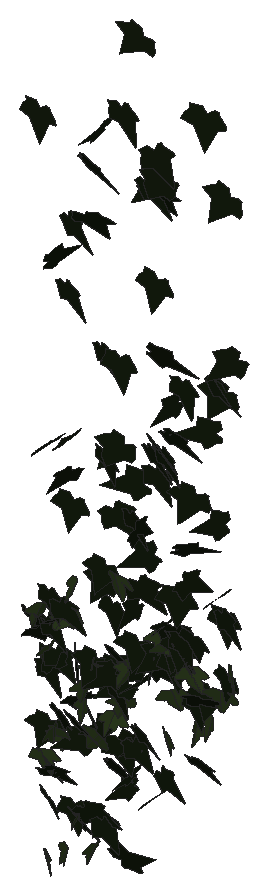
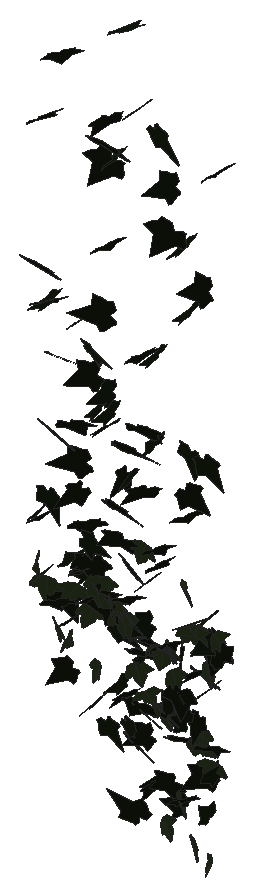
# SketchUp Ruby script. Lengths in inches.
U = 1.inch
M = Sketchup.active_model
def pt(a) = Geom::Point3d.new(a.map { |v| v * U })
def face(e, loops, mat)
  f = e.add_face(loops[0].map { |a| pt(a) })
  loops[1..].each { |l| e.add_face(l.map { |a| pt(a) }).erase! }
  f.material = f.back_material = mat if mat
  f
end
# faces: each face lists its corners as indices into pts; further lists are holes
def faces(e, pts, list, mat = nil) = list.each { |f| face(e, (f[0].is_a?(Array) ? f : [f]).map { |l| l.map { |i| pts[i] } }, mat) }
# xy, xz, yz: faces in a plane at the given z, y or x. An outline is a flat list of corners, or four numbers for a rectangle; further outlines are holes
def ring(l) = l.size == 4 ? [[l[0], l[1]], [l[2], l[1]], [l[2], l[3]], [l[0], l[3]]] : l.each_slice(2).to_a
def flat(e, list, mat, &to3) = list.each { |f| face(e, (f[0].is_a?(Array) ? f : [f]).map { |l| ring(l).map { |u, v| to3.(u, v) } }, mat) }
def xy(e, z, list, mat = nil) = flat(e, list, mat) { |x, y| [x, y, z] }
def xz(e, y, list, mat = nil) = flat(e, list, mat) { |x, z| [x, y, z] }
def yz(e, x, list, mat = nil) = flat(e, list, mat) { |y, z| [x, y, z] }
def lines(e, pts, list) = list.each { |a, b| e.add_line(pt(pts[a]), pt(pts[b])) }
# prism: a flat outline (further loops are holes) pulled along v
def prism(e, loops, v, mat = nil)
  f = face(e, loops, mat); d = Geom::Vector3d.new(v.map { |x| x * U })
  f.pushpull(f.normal.samedirection?(d) ? d.length : -d.length)
end
def box(e, o, s, mat = nil) = prism(e, [[o, [o[0] + s[0], o[1], o[2]], [o[0] + s[0], o[1] + s[1], o[2]], [o[0], o[1] + s[1], o[2]]]], [0, 0, s[2]], mat)
def at(x, y, z, deg = 0) = Geom::Transformation.translation(pt([x, y, z])) * Geom::Transformation.rotation(ORIGIN, Z_AXIS, deg.degrees)
def axes(o, x, y, z) = Geom::Transformation.new([*x, 0, *y, 0, *z, 0, *pt(o).to_a, 1])
def part(name) = M.definitions.add(name)
# library, detail: a bought-in or finely detailed component or shape, given as its bounding box
def library(name, o, s) = part(name).tap { |d| box(d.entities, o, s) }
def detail(e, o, s) = box(e.add_group.entities, o, s)
def put(e, d, t, mat = nil) = e.add_instance(d, t).tap { |i| i.material = mat if mat }
def group(e, t, mat = nil) = e.add_group.tap { |g| g.transformation = t; g.material = mat if mat }.entities
root = M.entities
M.materials.add("1026 AP 7946 SUNNY SIDE UP").color = [254, 231, 186]
M.materials.add("efeu1").color = [18, 25, 13]
M.materials.add("efeu2").color = [43, 57, 29]
c1 = part("ivyleaf_9")
p = [[1.54,2.16,1.25],[1.36,2.04,1.19],[-0.21,0.99,0.68],[-0.71,1.11,0.82],[-0.85,0.86,0.67],[-0.8,0.17,0.21],
  [-0.9,-0.01,0.1],[-0.67,-0.16,-0.02],[-0.08,-0.08,-0.05],[-0.03,-0.6,-0.4],[0.65,-0.88,-0.66],[0.83,-0.6,-0.49],
  [1.29,-0.42,-0.43],[1.8125,-0.07,-0.26],[1.21,0.44,0.15]]
faces(c1.entities,p,[[0,1,2,3,4,5,6,7,8,9,10,11,12,13,14]],"efeu1")
c2 = part("ivyleaf_10")
p = [[0,0.5,-0.03],[-0.0625,2.02,-0.43],[-0.19,2.01,-0.46],[-0.54,1.05,-0.29],[-0.52,0.625,-0.18],[-0.83,0.76,-0.28],
  [-1.16,0.64,-0.33],[-1.15,0.33,-0.24],[-0.77,-0.39,0.02],[-0.3,-0.51,0.16],[0.04,-0.48,0.23],[-0.02,2.01,-0.4375],
  [-0.06,2.01,-0.43],[0.04,-0.49,0.23],[0.67,-0.49,0.14],[1.38,0.36,-0.2],[1.375,0.51,-0.24],[0.81,0.65,-0.19],
  [0.62,0.59,-0.15],[0.6,1.09,-0.28],[0.5,1.23,-0.31]]
faces(c2.entities,p,[[0,1,2,3,4,5,6,7,8,9,10],[11,12,0,13,14,15,16,17,18,19,20]],"efeu2")
put(root,c1,axes([152.38,212.64,301.87],[0.59267,-0.16928,-0.16841],[0.27344,-0.00496,0.4208],[-0.24775,-0.41043,0.06156]),"1026 AP 7946 SUNNY SIDE UP")
put(root,c2,axes([152.84,212.47,302.625],[-0.0681,-0.36984,0.14423],[0.05239,-0.14585,-0.38143],[0.62079,-0.02827,0.04802]),"1026 AP 7946 SUNNY SIDE UP")
put(root,c1,axes([152.77,212.59,324.46],[-0.08062,-0.44601,0.10628],[-0.00062,-0.10632,-0.46298],[0.72074,-0.04998,0.01149]),"1026 AP 7946 SUNNY SIDE UP")
put(root,c1,axes([153.01,212.125,301.88],[0.28925,0.3534,-0.00163],[0.01988,-0.01062,-0.41016],[-0.55536,0.18368,-0.01553]),"1026 AP 7946 SUNNY SIDE UP")
put(root,c1,axes([153.09,212.79,297.5625],[-0.42227,-0.2678,-0.03495],[0.09587,-0.01572,-0.38682],[0.41319,-0.27004,0.05404]),"1026 AP 7946 SUNNY SIDE UP")
put(root,c2,axes([153.31,212.47,301.09],[-0.02165,-0.39705,-0.05057],[-0.01728,0.04722,-0.4088],[0.62841,-0.01238,-0.01298]),"1026 AP 7946 SUNNY SIDE UP")
put(root,c1,axes([152.97,212.4,296.27],[0.48845,-0.20747,0.00156],[-0.02814,-0.03161,-0.3832],[0.32504,0.30904,-0.03551]),"1026 AP 7946 SUNNY SIDE UP")
put(root,c2,axes([153.21,212.26,296.44],[-0.55173,-0.04794,-0.1243],[0.20286,-0.09686,-0.34822],[0.01899,-0.35809,0.10854]),"1026 AP 7946 SUNNY SIDE UP")
put(root,c1,axes([153.68,212.25,300.45],[0.063,0.26432,0.3021],[-0.32917,0.26266,-0.21399],[-0.52424,-0.13316,0.17067]),"1026 AP 7946 SUNNY SIDE UP")
put(root,c1,axes([153.24,212.17,302.16],[0.36825,0.22617,0.24006],[0.15081,0.22472,-0.32447],[-0.48632,0.24094,0.08116]),"1026 AP 7946 SUNNY SIDE UP")
put(root,c1,axes([153.14,212.54,300.19],[0.16246,-0.37821,-0.06989],[-0.02092,0.06446,-0.40351],[0.60324,0.10409,0.00483]),"1026 AP 7946 SUNNY SIDE UP")
put(root,c2,axes([153.25,212.41,291.94],[-0.17561,0.2896,-0.20904],[0.11283,-0.19156,-0.32088],[-0.54597,-0.13274,0.00092]),"1026 AP 7946 SUNNY SIDE UP")
put(root,c1,axes([153.09,212.7,294.28],[0.1363,-0.25992,0.25879],[0.11096,-0.24273,-0.28358],[0.55908,0.11154,-0.00681]),"1026 AP 7946 SUNNY SIDE UP")
put(root,c1,axes([153.75,212.1,310.41],[-0.20385,0.36682,-0.15139],[0.01655,-0.15357,-0.39973],[-0.62235,-0.12423,0.03896]),"1026 AP 7946 SUNNY SIDE UP")
put(root,c1,axes([153.25,212.57,303.38],[0.1275,-0.39729,0.03992],[0.00004,-0.04184,-0.41788],[0.62801,0.08066,-0.00808]),"1026 AP 7946 SUNNY SIDE UP")
put(root,c2,axes([153.99,212.48,297.3125],[0.17742,0.01833,-0.37186],[-0.54367,0.11597,-0.10457],[0.16608,0.36007,0.05494]),"1026 AP 7946 SUNNY SIDE UP")
put(root,c2,axes([153.67,212.24,297.66],[0.00859,-0.36437,-0.12292],[0.04841,0.1173,-0.37337],[0.59992,-0.00425,0.03189]),"1026 AP 7946 SUNNY SIDE UP")
put(root,c1,axes([153.41,212.34,302.31],[0.23614,-0.36549,-0.1104],[-0.04561,0.10165,-0.4063],[0.59624,0.15252,0.01264]),"1026 AP 7946 SUNNY SIDE UP")
put(root,c2,axes([154.05,212.66,302.59],[-0.45612,-0.10984,0.25829],[-0.31335,-0.16698,-0.31309],[0.29637,-0.3456,0.06648]),"1026 AP 7946 SUNNY SIDE UP")
put(root,c1,axes([153.47,212.2,295.85],[0.53767,0.11655,0.09473],[0.14103,0.01971,-0.37191],[-0.1852,0.35337,-0.0082]),"1026 AP 7946 SUNNY SIDE UP")
put(root,c1,axes([153.57,212.62,300.88],[0.07856,-0.36003,-0.16441],[0.07557,0.16322,-0.3676],[0.61331,0.026,0.06635]),"1026 AP 7946 SUNNY SIDE UP")
put(root,c1,axes([153.85,212.38,298.45],[0.46288,-0.05409,-0.24683],[-0.37445,0.02679,-0.30789],[0.09267,0.37841,-0.01122]),"1026 AP 7946 SUNNY SIDE UP")
put(root,c1,axes([153.71,212.05,318.36],[0.19098,0.13648,0.44339],[0.43001,0.3314,-0.18617],[-0.56347,0.29917,0.00821]),"1026 AP 7946 SUNNY SIDE UP")
put(root,c2,axes([154.01,212.7,302.73],[0.46112,0.20838,-0.17692],[-0.21603,-0.10516,-0.37119],[-0.36691,0.3238,-0.00381]),"1026 AP 7946 SUNNY SIDE UP")
put(root,c1,axes([154.28,212.6,309.05],[-0.12867,0.23577,-0.34477],[0.09364,-0.33218,-0.257],[-0.6386,-0.09621,0.03178]),"1026 AP 7946 SUNNY SIDE UP")
put(root,c1,axes([153.81,212.61,303.05],[0.20145,-0.36895,-0.1118],[0.13513,0.1369,-0.38153],[0.58847,0.09487,0.12589]),"1026 AP 7946 SUNNY SIDE UP")
put(root,c1,axes([154.42,212.17,310.63],[-0.01495,0.39155,0.1484],[-0.04266,0.14098,-0.40202],[-0.65344,-0.01816,0.02285]),"1026 AP 7946 SUNNY SIDE UP")
put(root,c2,axes([154.27,212.24,292.54],[0.31163,-0.30663,-0.12815],[-0.06241,0.11989,-0.37415],[0.51552,0.19987,0.03217]),"1026 AP 7946 SUNNY SIDE UP")
put(root,c1,axes([154.41,212.58,307.82],[-0.20704,-0.39674,0.03588],[0.01254,-0.04167,-0.43036],[0.62642,-0.13029,0.02047]),"1026 AP 7946 SUNNY SIDE UP")
put(root,c2,axes([154.56,212.41,304.3125],[0.34317,-0.33521,0.05099],[0.01585,-0.05468,-0.41181],[0.53301,0.21744,-0.02058]),"1026 AP 7946 SUNNY SIDE UP")
put(root,c1,axes([154.89,212.76,297.38],[-0.53413,-0.04392,0.15932],[-0.21018,-0.12468,-0.33913],[0.14113,-0.3519,0.09792]),"1026 AP 7946 SUNNY SIDE UP")
put(root,c1,axes([154.31,212.3,317.32],[0.29807,-0.40567,-0.02063],[-0.01776,0.01429,-0.4612],[0.63824,0.18986,-0.0032]),"1026 AP 7946 SUNNY SIDE UP")
put(root,c1,axes([154.76,212.4,299.4],[0.1908,0.36177,-0.05805],[-0.01768,-0.05781,-0.39336],[-0.57595,0.12163,-0.00716]),"1026 AP 7946 SUNNY SIDE UP")
put(root,c1,axes([154.53,212.57,294.51],[-0.13958,-0.36139,-0.05306],[0.06952,0.03986,-0.38161],[0.56931,-0.09347,0.03359]),"1026 AP 7946 SUNNY SIDE UP")
put(root,c2,axes([154.88,212.3125,294.35],[0.19913,-0.36578,-0.02964],[-0.03252,0.02108,-0.39843],[0.57577,0.12769,-0.01225]),"1026 AP 7946 SUNNY SIDE UP")
put(root,c1,axes([154.54,212.23,320.38],[0.36438,-0.37295,-0.11547],[-0.07791,0.09865,-0.45165],[0.6064,0.23677,0.01136]),"1026 AP 7946 SUNNY SIDE UP")
put(root,c1,axes([154.42,212.55,298.17],[0.30568,-0.23065,0.25573],[0.24997,-0.19237,-0.31188],[0.47225,0.25112,-0.00045]),"1026 AP 7946 SUNNY SIDE UP")
put(root,c1,axes([155.13,211.96,300.62],[0.02326,-0.17869,0.38061],[0.07286,0.36908,0.18365],[-0.64264,0.03538,0.03459]),"1026 AP 7946 SUNNY SIDE UP")
put(root,c2,axes([155.13,212.41,300.09],[-0.15595,-0.38043,0.04045],[0.04749,-0.05044,-0.40302],[0.59984,-0.09491,0.04242]),"1026 AP 7946 SUNNY SIDE UP")
put(root,c1,axes([154.68,212.41,294.07],[0.32696,-0.21165,0.23496],[0.21462,-0.18606,-0.30556],[0.4412,0.24736,-0.02548]),"1026 AP 7946 SUNNY SIDE UP")
put(root,c2,axes([155.04,212.35,299.26],[0.42752,-0.25383,0.10768],[0.15285,-0.05071,-0.38238],[0.40459,0.28737,0.03068]),"1026 AP 7946 SUNNY SIDE UP")
put(root,c1,axes([155.19,212.74,298.46],[0.01744,-0.11246,0.37505],[0.09769,-0.35945,-0.11824],[0.5921,0.06262,0.00846]),"1026 AP 7946 SUNNY SIDE UP")
put(root,c2,axes([155.52,212.48,293.0625],[0.01729,-0.38054,0.05601],[0.01268,-0.05631,-0.39247],[0.60479,0.01206,0.00663]),"1026 AP 7946 SUNNY SIDE UP")
put(root,c2,axes([155.37,212.41,301.18],[0.38105,-0.27614,0.161],[0.14727,-0.12769,-0.37901],[0.47796,0.2595,-0.01158]),"1026 AP 7946 SUNNY SIDE UP")
put(root,c1,axes([155.04,212.5625,323],[0.6375,-0.20175,0.08183],[0.08669,-0.06947,-0.46537],[0.33041,0.40748,-0.03578]),"1026 AP 7946 SUNNY SIDE UP")
put(root,c1,axes([155.28,212.32,320.75],[0.65941,0.18642,-0.0309],[-0.01909,-0.04885,-0.47131],[-0.29655,0.41767,-0.03836]),"1026 AP 7946 SUNNY SIDE UP")
put(root,c2,axes([155.92,212.1875,298.12],[-0.51022,0.07138,0.23066],[-0.35739,-0.00105,-0.33961],[-0.09149,-0.394,0.04031]),"1026 AP 7946 SUNNY SIDE UP")
put(root,c1,axes([155.61,212.49,301.29],[-0.31678,-0.35493,0.10209],[-0.04692,-0.09916,-0.42039],[0.57839,-0.20243,0.02181]),"1026 AP 7946 SUNNY SIDE UP")
put(root,c2,axes([155.78,212.41,300.99],[-0.59877,-0.12399,0.01024],[0.00379,-0.0416,-0.41072],[0.19565,-0.37867,0.03929]),"1026 AP 7946 SUNNY SIDE UP")
put(root,c1,axes([156.11,212.52,298.51],[-0.48896,0.21647,0.04515],[-0.07,0.01054,-0.38989],[-0.33977,-0.31369,0.01535]),"1026 AP 7946 SUNNY SIDE UP")
put(root,c1,axes([155.42,212.13,294.85],[0.02672,-0.00234,-0.39553],[0.37231,0.30258,0.01066],[0.47522,-0.23692,0.01389]),"1026 AP 7946 SUNNY SIDE UP")
put(root,c1,axes([156.24,212.15,325],[-0.38818,0.37554,-0.11417],[0.07073,-0.10547,-0.46315],[-0.61256,-0.25016,0.01887]),"1026 AP 7946 SUNNY SIDE UP")
put(root,c1,axes([155.97,212.55,304.93],[-0.21781,-0.33573,0.19638],[-0.09672,-0.1828,-0.37503],[0.60081,-0.15114,0.01082]),"1026 AP 7946 SUNNY SIDE UP")
put(root,c1,axes([155.78,212.67,314.92],[0.30272,-0.38907,-0.01006],[-0.02408,0.00085,-0.44698],[0.61141,0.19266,-0.01262]),"1026 AP 7946 SUNNY SIDE UP")
put(root,c1,axes([156.125,212.43,305.59],[-0.28187,-0.35596,0.08899],[-0.02341,-0.09125,-0.41017],[0.57624,-0.17783,0.02686]),"1026 AP 7946 SUNNY SIDE UP")
put(root,c2,axes([156.3125,212.68,298.95],[0.33906,0.27536,-0.17531],[-0.14241,-0.14693,-0.36072],[-0.49,0.23324,-0.01647]),"1026 AP 7946 SUNNY SIDE UP")
put(root,c1,axes([156.61,212.3125,301.1],[-0.6145,-0.00765,0.03466],[-0.05151,-0.03944,-0.40093],[0.01726,-0.39026,0.03754]),"1026 AP 7946 SUNNY SIDE UP")
put(root,c1,axes([156.41,212.72,301.25],[-0.54212,-0.17249,-0.08893],[0.20843,-0.08591,-0.3733],[0.21937,-0.34463,0.13492]),"1026 AP 7946 SUNNY SIDE UP")
put(root,c1,axes([156.24,212.15,294.53],[0.0982,-0.35578,-0.2196],[-0.0837,0.20485,-0.37062],[0.64512,0.08073,-0.01466]),"1026 AP 7946 SUNNY SIDE UP")
put(root,c1,axes([156.15,212.42,310.45],[0.12462,-0.3783,0.17271],[0.04712,-0.1672,-0.39913],[0.65031,0.08461,-0.00418]),"1026 AP 7946 SUNNY SIDE UP")
put(root,c1,axes([156.28,212.59,296.92],[0.5643,-0.11985,0.04953],[0.0551,-0.04836,-0.38845],[0.19584,0.35893,-0.03343]),"1026 AP 7946 SUNNY SIDE UP")
put(root,c1,axes([156.44,212.49,303.99],[0.0253,-0.39694,0.08706],[-0.00664,-0.08699,-0.40969],[0.63884,0.01481,-0.00771]),"1026 AP 7946 SUNNY SIDE UP")
put(root,c1,axes([156.84,212.58,311.13],[-0.62577,-0.15357,-0.01147],[0.03703,-0.03264,-0.43781],[0.23916,-0.39676,0.03778]),"1026 AP 7946 SUNNY SIDE UP")
put(root,c1,axes([157.1,212.52,298.04],[-0.39398,0.25,0.14966],[-0.20948,0.06871,-0.36164],[-0.40226,-0.28063,0.04175]),"1026 AP 7946 SUNNY SIDE UP")
put(root,c1,axes([156.98,212.61,300.64],[-0.57695,-0.08204,0.09754],[-0.11973,-0.08838,-0.38155],[0.15711,-0.36861,0.06739]),"1026 AP 7946 SUNNY SIDE UP")
put(root,c1,axes([156.5625,212.77,314.71],[-0.07514,-0.43164,-0.01289],[0.00649,0.00966,-0.44732],[0.67887,-0.04787,0.00285]),"1026 AP 7946 SUNNY SIDE UP")
put(root,c1,axes([156.44,212.41,302],[0.58229,-0.16012,-0.01614],[-0.04252,-0.02549,-0.41429],[0.24924,0.36973,-0.03297]),"1026 AP 7946 SUNNY SIDE UP")
put(root,c2,axes([156.91,212.64,299.87],[-0.32214,-0.3101,0.09578],[-0.03233,-0.09941,-0.38162],[0.50883,-0.20264,0.03639]),"1026 AP 7946 SUNNY SIDE UP")
put(root,c2,axes([156.86,212.26,305.37],[-0.60547,0.10544,-0.05747],[0.05303,-0.08662,-0.40468],[-0.18037,-0.3794,0.07392]),"1026 AP 7946 SUNNY SIDE UP")
put(root,c1,axes([156.6,212.41,308.25],[0.06816,-0.29063,-0.32088],[0.0867,0.31265,-0.29236],[0.66231,-0.01102,0.07129]),"1026 AP 7946 SUNNY SIDE UP")
put(root,c1,axes([156.61,212.45,300.41],[0.19777,-0.36955,0.08059],[0.01527,-0.08146,-0.40226],[0.59446,0.12504,-0.01648]),"1026 AP 7946 SUNNY SIDE UP")
put(root,c1,axes([157.41,212.48,296.36],[-0.52203,0.18429,-0.04604],[0.03731,-0.05115,-0.39],[-0.29623,-0.33121,0.03203]),"1026 AP 7946 SUNNY SIDE UP")
put(root,c1,axes([156.91,212.44,298.12],[-0.3345,-0.19543,-0.29831],[0.41263,0.13246,-0.29105],[0.3604,-0.33304,0.05636]),"1026 AP 7946 SUNNY SIDE UP")
put(root,c1,axes([156.91,212.46,325.96],[0.13992,-0.45923,-0.00836],[0.02101,0.0082,-0.48161],[0.72184,0.08878,0.01564]),"1026 AP 7946 SUNNY SIDE UP")
put(root,c2,axes([157.27,212.42,301.52],[-0.11228,-0.29504,0.27349],[0.05887,-0.27519,-0.30439],[0.62307,-0.02717,0.07805]),"1026 AP 7946 SUNNY SIDE UP")
put(root,c1,axes([157.55,212.41,296.97],[-0.37803,0.26796,-0.13267],[0.09572,-0.11973,-0.37005],[-0.45863,-0.24585,0.03212]),"1026 AP 7946 SUNNY SIDE UP")
put(root,c1,axes([156.91,212.55,292.93],[0.00973,-0.04424,0.42692],[0.55916,-0.21605,-0.03048],[0.3425,0.35399,0.03763]),"1026 AP 7946 SUNNY SIDE UP")
put(root,c1,axes([157.91,212.46,309.83],[-0.57876,0.10107,0.1991],[-0.32236,-0.0342,-0.38514],[-0.11465,-0.41405,0.07783]),"1026 AP 7946 SUNNY SIDE UP")
put(root,c1,axes([158,212.2,301.89],[-0.26425,-0.01081,-0.36542],[-0.55548,0.04171,0.17139],[0.05205,0.39023,-0.02613]),"1026 AP 7946 SUNNY SIDE UP")
put(root,c1,axes([157.6875,212.38,304.45],[-0.52579,0.11472,-0.20606],[0.27297,-0.10837,-0.36247],[-0.23997,-0.37462,0.03917]),"1026 AP 7946 SUNNY SIDE UP")
put(root,c2,axes([157.76,212.5,301.88],[-0.4976,-0.23901,0.05995],[-0.03706,-0.06713,-0.40697],[0.38553,-0.31494,0.03826]),"1026 AP 7946 SUNNY SIDE UP")
put(root,c1,axes([157.76,212.62,329.37],[-0.44588,-0.27501,0.27597],[-0.01805,-0.32845,-0.35972],[0.60511,-0.21244,0.19262]),"1026 AP 7946 SUNNY SIDE UP")
put(root,c1,axes([157.7,212.48,302.78],[-0.31133,-0.35577,0.01218],[0.0815,-0.04447,-0.41401],[0.55387,-0.19343,0.06777]),"1026 AP 7946 SUNNY SIDE UP")
put(root,c1,axes([157.51,212.29,308.35],[0.26017,-0.3802,0.02003],[-0.0077,-0.02567,-0.42705],[0.59875,0.16487,-0.0142]),"1026 AP 7946 SUNNY SIDE UP")
put(root,c1,axes([157.58,212.37,298.33],[0.13237,-0.32693,-0.18945],[-0.00513,0.18594,-0.34448],[0.58836,0.07517,0.03962]),"1026 AP 7946 SUNNY SIDE UP")
put(root,c1,axes([158.1,212.47,301.33],[-0.36656,0.24596,-0.19155],[0.0528,-0.21309,-0.33252],[-0.48328,-0.20984,0.10896]),"1026 AP 7946 SUNNY SIDE UP")
put(root,c1,axes([157.61,212.51,298.89],[0.40221,-0.28478,-0.02993],[-0.0139,0.02891,-0.39396],[0.44965,0.25563,0.01459]),"1026 AP 7946 SUNNY SIDE UP")
put(root,c1,axes([158.44,212.38,306.92],[-0.63083,0.07826,0.0655],[-0.1062,-0.01736,-0.42009],[-0.11713,-0.40575,0.02814]),"1026 AP 7946 SUNNY SIDE UP")
put(root,c1,axes([158.11,211.83,308.17],[0.01407,0.01299,-0.43199],[-0.35844,0.35235,0.00829],[0.55394,0.22767,0.01634]),"1026 AP 7946 SUNNY SIDE UP")
put(root,c1,axes([157.84,212.375,305.48],[-0.09097,-0.18868,-0.37341],[0.45024,0.24102,-0.17545],[0.45631,-0.27543,0.09867]),"1026 AP 7946 SUNNY SIDE UP")
put(root,c2,axes([158.3125,212.52,302.32],[0.60402,-0.03418,-0.11875],[-0.16496,0.09193,-0.38837],[0.09174,0.39032,0.0835]),"1026 AP 7946 SUNNY SIDE UP")
put(root,c1,axes([158.28,212.59,302.31],[-0.13859,-0.04269,-0.39374],[0.53088,-0.19584,-0.05886],[-0.28876,-0.33957,0.08076]),"1026 AP 7946 SUNNY SIDE UP")
put(root,c1,axes([158.76,212.23,296.49],[-0.19542,0.34331,-0.12183],[0.02989,-0.12073,-0.37615],[-0.57117,-0.12378,0.022]),"1026 AP 7946 SUNNY SIDE UP")
put(root,c1,axes([158.2,212.55,311.38],[0.40827,-0.33735,-0.01285],[-0.02768,-0.00023,-0.43831],[0.52998,0.25986,-0.01299]),"1026 AP 7946 SUNNY SIDE UP")
put(root,c1,axes([158.23,212.34,323.19],[0.35209,-0.39865,-0.09879],[-0.00736,0.10421,-0.46804],[0.64385,0.21919,0.04867]),"1026 AP 7946 SUNNY SIDE UP")
put(root,c1,axes([158.47,212.34,322.96],[0.69881,0.14006,-0.04441],[-0.04586,-0.05293,-0.47844],[-0.2262,0.44343,-0.04019]),"1026 AP 7946 SUNNY SIDE UP")
put(root,c1,axes([158.62,212.5,318.99],[-0.17198,-0.42874,0.10071],[-0.02703,-0.099,-0.45635],[0.69179,-0.11045,0.00721]),"1026 AP 7946 SUNNY SIDE UP")
put(root,c1,axes([158.98,212.55,302.62],[-0.55562,-0.16703,0.1109],[-0.1275,-0.0814,-0.40127],[0.28615,-0.3606,0.03654]),"1026 AP 7946 SUNNY SIDE UP")
put(root,c1,axes([158.25,212.57,302.08],[0.18402,-0.0341,-0.42151],[0.63421,0.08798,0.11186],[0.119,-0.41617,0.05562]),"1026 AP 7946 SUNNY SIDE UP")
put(root,c1,axes([158.54,212.5,310.58],[0.11632,-0.40754,-0.09449],[0.01376,0.0923,-0.42542],[0.65592,0.07034,0.02568]),"1026 AP 7946 SUNNY SIDE UP")
put(root,c2,axes([158.8125,212.68,303.32],[-0.50433,-0.24124,0.02681],[0.11901,-0.14247,-0.38046],[0.36274,-0.28866,0.1621]),"1026 AP 7946 SUNNY SIDE UP")
put(root,c1,axes([159.14,212.36,323.63],[-0.73675,-0.01922,-0.01718],[0.03065,-0.07648,-0.47696],[0.02555,-0.46256,0.07679]),"1026 AP 7946 SUNNY SIDE UP")
put(root,c2,axes([158.95,212.65,302.99],[-0.24676,-0.37071,0.00866],[0.02574,-0.01832,-0.41419],[0.58257,-0.15621,0.02196]),"1026 AP 7946 SUNNY SIDE UP")
put(root,c1,axes([158.54,212.26,312.04],[0.53287,-0.27516,-0.00641],[-0.03673,-0.0214,-0.44868],[0.43117,0.33825,-0.0303]),"1026 AP 7946 SUNNY SIDE UP")
put(root,c1,axes([158.72,212.23,324.81],[0.07033,-0.39373,-0.2541],[-0.03798,0.24324,-0.40679],[0.7277,0.05075,0.00333]),"1026 AP 7946 SUNNY SIDE UP")
put(root,c2,axes([159.02,212.53,299.15],[-0.39126,0.29496,-0.01745],[-0.01513,-0.0324,-0.39667],[-0.46447,-0.24741,0.02762]),"1026 AP 7946 SUNNY SIDE UP")
put(root,c1,axes([158.74,212.67,311.41],[0.29336,-0.38618,0.00701],[-0.02566,-0.01786,-0.44134],[0.60686,0.18593,-0.02205]),"1026 AP 7946 SUNNY SIDE UP")
put(root,c1,axes([158.52,212.48,315.76],[0.59346,-0.07404,0.26818],[0.37922,-0.11227,-0.39314],[0.19452,0.44478,-0.05176]),"1026 AP 7946 SUNNY SIDE UP")
put(root,c1,axes([159.35,212.51,304.01],[0.31439,0.25884,-0.25489],[-0.19425,-0.2179,-0.33697],[-0.53017,0.23333,-0.02769]),"1026 AP 7946 SUNNY SIDE UP")
put(root,c1,axes([159.0625,212.28,297.53],[0.3188,-0.28809,-0.19621],[-0.11517,0.17804,-0.35981],[0.52923,0.21228,0.03989]),"1026 AP 7946 SUNNY SIDE UP")
put(root,c1,axes([159.53,212.54,313.91],[-0.57525,0.12637,-0.19239],[0.21607,-0.15888,-0.38753],[-0.2823,-0.37913,0.09542]),"1026 AP 7946 SUNNY SIDE UP")
put(root,c1,axes([159.24,212.69,302.4],[-0.03823,-0.39675,-0.00041],[0.02526,-0.00284,-0.40917],[0.62335,-0.02422,0.01656]),"1026 AP 7946 SUNNY SIDE UP")
put(root,c1,axes([159.76,212.38,304.78],[-0.39922,0.15482,-0.29459],[0.20972,-0.2824,-0.28031],[-0.46766,-0.25881,0.12577]),"1026 AP 7946 SUNNY SIDE UP")
put(root,c2,axes([159.67,212.11,301.4],[-0.42721,-0.25317,-0.12718],[0.18299,0.05313,-0.38021],[0.40224,-0.29305,0.03789]),"1026 AP 7946 SUNNY SIDE UP")
put(root,c1,axes([159.35,212.28,312.57],[0.64722,-0.06906,0.08977],[0.12126,-0.06544,-0.42717],[0.12662,0.4157,-0.04978]),"1026 AP 7946 SUNNY SIDE UP")
put(root,c1,axes([159.42,212.52,303.5],[0.35591,-0.35219,0.10248],[0.0644,-0.09422,-0.43153],[0.57271,0.22946,-0.01516]),"1026 AP 7946 SUNNY SIDE UP")
put(root,c1,axes([159.73,212.43,305.6],[-0.29996,-0.36828,-0.08153],[0.06184,0.0664,-0.42686],[0.58838,-0.19473,0.0033]),"1026 AP 7946 SUNNY SIDE UP")
put(root,c1,axes([159.74,212.55,303.4],[-0.22118,-0.36898,0.03926],[0.06444,-0.05817,-0.40263],[0.58006,-0.13423,0.0597]),"1026 AP 7946 SUNNY SIDE UP")
put(root,c1,axes([159.85,212.41,303.7],[0.10156,-0.40658,-0.0116],[-0.00693,0.00837,-0.42404],[0.63942,0.06467,-0.00275]),"1026 AP 7946 SUNNY SIDE UP")
put(root,c1,axes([160.01,212.32,315],[0.08145,-0.43253,0.00846],[-0.00696,-0.01127,-0.4488],[0.68028,0.05167,-0.0056]),"1026 AP 7946 SUNNY SIDE UP")
put(root,c1,axes([160.36,212.61,310.13],[-0.49419,-0.28611,-0.00544],[0.03403,-0.01835,-0.43699],[0.44863,-0.31378,0.02715]),"1026 AP 7946 SUNNY SIDE UP")
put(root,c2,axes([160.23,212.47,302.375],[-0.51593,-0.13628,-0.16762],[0.31046,-0.08949,-0.33508],[0.11988,-0.35479,0.14639]),"1026 AP 7946 SUNNY SIDE UP")
put(root,c1,axes([160.23,212.71,303.79],[-0.01975,-0.35169,0.19244],[0.13063,-0.18706,-0.35437],[0.6139,0.02849,0.08159]),"1026 AP 7946 SUNNY SIDE UP")
put(root,c1,axes([160.3,212.77,301],[0.0151,-0.39045,0.0397],[0.00011,-0.04076,-0.4026],[0.61728,0.00956,-0.0009]),"1026 AP 7946 SUNNY SIDE UP")
put(root,c2,axes([160.47,212.66,300],[-0.00622,0.29362,-0.26698],[-0.04569,-0.26034,-0.30299],[-0.61584,0.01635,0.02518]),"1026 AP 7946 SUNNY SIDE UP")
put(root,c1,axes([160.43,211.91,306.6875],[0.08003,-0.01907,-0.43564],[-0.16417,0.41208,-0.02969],[0.64486,0.10727,0.04651]),"1026 AP 7946 SUNNY SIDE UP")
put(root,c1,axes([160.23,211.9,308],[0.4373,0.0813,0.31803],[0.41741,0.16742,-0.29126],[-0.27754,0.37991,0.06305]),"1026 AP 7946 SUNNY SIDE UP")
put(root,c1,axes([161.1875,212.72,313.07],[-0.6004,0.13826,0.14798],[-0.28581,-0.1175,-0.38405],[-0.12662,-0.39039,0.16522]),"1026 AP 7946 SUNNY SIDE UP")
put(root,c1,axes([160.46,212.49,298.56],[0.60849,-0.03557,-0.024],[-0.03652,-0.00035,-0.40034],[0.0558,0.38767,-0.00028]),"1026 AP 7946 SUNNY SIDE UP")
put(root,c1,axes([161.18,212.07,301.67],[0.16712,0.30376,-0.23297],[-0.33126,-0.14969,-0.30768],[-0.49676,0.20201,0.1268]),"1026 AP 7946 SUNNY SIDE UP")
put(root,c1,axes([161,212.78,301.64],[-0.33349,-0.33131,-0.03064],[0.06597,0.00611,-0.40388],[0.51861,-0.21382,0.03168]),"1026 AP 7946 SUNNY SIDE UP")
put(root,c2,axes([161.02,212.68,300.43],[0.41612,-0.2748,0.10121],[0.11862,-0.06588,-0.39332],[0.44415,0.27506,0.01022]),"1026 AP 7946 SUNNY SIDE UP")
put(root,c1,axes([161.04,212.48,327.13],[-0.24148,-0.45065,-0.02249],[0.03461,0.01285,-0.49009],[0.7084,-0.15425,0.01628]),"1026 AP 7946 SUNNY SIDE UP")
put(root,c1,axes([161.89,212.43,309.4375],[-0.55816,0.20796,0.07649],[-0.12182,0.01196,-0.42274],[-0.32448,-0.36221,0.02714]),"1026 AP 7946 SUNNY SIDE UP")
put(root,c1,axes([161.76,212.32,306.23],[-0.11486,0.41114,-0.00642],[-0.00751,-0.00955,-0.43019],[-0.64657,-0.07293,0.00614]),"1026 AP 7946 SUNNY SIDE UP")
put(root,c1,axes([161.43,212.52,315.51],[0.38108,-0.36728,-0.0647],[0.00933,0.07625,-0.45034],[0.58528,0.23793,0.0493]),"1026 AP 7946 SUNNY SIDE UP")
put(root,c2,axes([161.91,212.3125,302.04],[-0.60047,-0.0909,0.02468],[-0.02497,-0.03858,-0.40312],[0.14589,-0.38071,0.03258]),"1026 AP 7946 SUNNY SIDE UP")
put(root,c1,axes([161.88,212.48,315.22],[-0.38019,-0.34606,0.13942],[0.01405,-0.16906,-0.42376],[0.58524,-0.22076,0.10074]),"1026 AP 7946 SUNNY SIDE UP")
put(root,c1,axes([161.78,212.85,302.53],[-0.0275,-0.3471,0.19053],[-0.02638,-0.18627,-0.35906],[0.61933,-0.02335,-0.00684]),"1026 AP 7946 SUNNY SIDE UP")
put(root,c1,axes([161.82,212.66,305.32],[-0.06582,-0.4064,0.04576],[0.02255,-0.0484,-0.42071],[0.64284,-0.03991,0.01945]),"1026 AP 7946 SUNNY SIDE UP")
put(root,c1,axes([162.04,212.6,323.79],[-0.3505,-0.35369,0.24298],[-0.09236,-0.24038,-0.42633],[0.66383,-0.22019,0.06898]),"1026 AP 7946 SUNNY SIDE UP")
put(root,c1,axes([161.98,212.33,305.53],[0.2733,-0.36617,-0.09652],[-0.08166,0.0767,-0.41688],[0.58788,0.18088,-0.01303]),"1026 AP 7946 SUNNY SIDE UP")
put(root,c1,axes([162.53,212.45,316.87],[-0.68704,-0.0144,-0.0381],[0.06143,-0.08891,-0.44128],[0.01032,-0.42938,0.09003]),"1026 AP 7946 SUNNY SIDE UP")
put(root,c2,axes([162.05,212.65,302.97],[0.19182,-0.25929,0.27818],[0.38189,-0.16318,-0.27392],[0.45014,0.24893,0.11385]),"1026 AP 7946 SUNNY SIDE UP")
